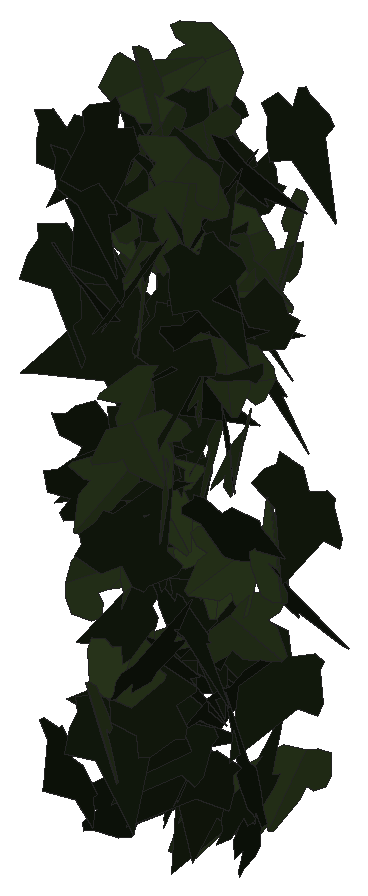
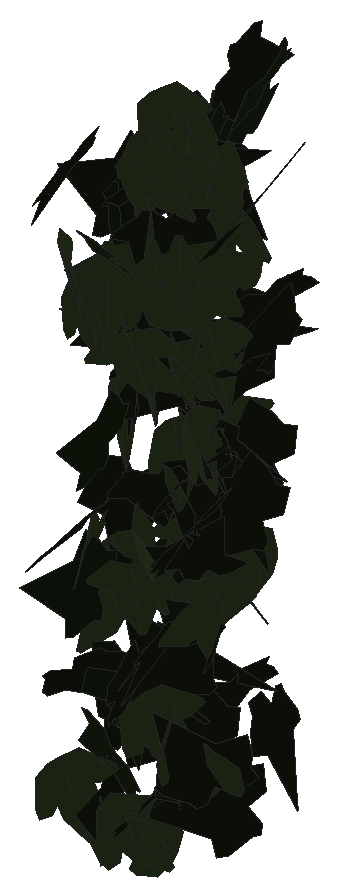
# SketchUp Ruby script. Lengths in inches.
U = 1.inch
M = Sketchup.active_model
def pt(a) = Geom::Point3d.new(a.map { |v| v * U })
def face(e, loops, mat)
  f = e.add_face(loops[0].map { |a| pt(a) })
  loops[1..].each { |l| e.add_face(l.map { |a| pt(a) }).erase! }
  f.material = f.back_material = mat if mat
  f
end
# faces: each face lists its corners as indices into pts; further lists are holes
def faces(e, pts, list, mat = nil) = list.each { |f| face(e, (f[0].is_a?(Array) ? f : [f]).map { |l| l.map { |i| pts[i] } }, mat) }
# xy, xz, yz: faces in a plane at the given z, y or x. An outline is a flat list of corners, or four numbers for a rectangle; further outlines are holes
def ring(l) = l.size == 4 ? [[l[0], l[1]], [l[2], l[1]], [l[2], l[3]], [l[0], l[3]]] : l.each_slice(2).to_a
def flat(e, list, mat, &to3) = list.each { |f| face(e, (f[0].is_a?(Array) ? f : [f]).map { |l| ring(l).map { |u, v| to3.(u, v) } }, mat) }
def xy(e, z, list, mat = nil) = flat(e, list, mat) { |x, y| [x, y, z] }
def xz(e, y, list, mat = nil) = flat(e, list, mat) { |x, z| [x, y, z] }
def yz(e, x, list, mat = nil) = flat(e, list, mat) { |y, z| [x, y, z] }
def lines(e, pts, list) = list.each { |a, b| e.add_line(pt(pts[a]), pt(pts[b])) }
# prism: a flat outline (further loops are holes) pulled along v
def prism(e, loops, v, mat = nil)
  f = face(e, loops, mat); d = Geom::Vector3d.new(v.map { |x| x * U })
  f.pushpull(f.normal.samedirection?(d) ? d.length : -d.length)
end
def box(e, o, s, mat = nil) = prism(e, [[o, [o[0] + s[0], o[1], o[2]], [o[0] + s[0], o[1] + s[1], o[2]], [o[0], o[1] + s[1], o[2]]]], [0, 0, s[2]], mat)
def at(x, y, z, deg = 0) = Geom::Transformation.translation(pt([x, y, z])) * Geom::Transformation.rotation(ORIGIN, Z_AXIS, deg.degrees)
def axes(o, x, y, z) = Geom::Transformation.new([*x, 0, *y, 0, *z, 0, *pt(o).to_a, 1])
def part(name) = M.definitions.add(name)
# library, detail: a bought-in or finely detailed component or shape, given as its bounding box
def library(name, o, s) = part(name).tap { |d| box(d.entities, o, s) }
def detail(e, o, s) = box(e.add_group.entities, o, s)
def put(e, d, t, mat = nil) = e.add_instance(d, t).tap { |i| i.material = mat if mat }
def group(e, t, mat = nil) = e.add_group.tap { |g| g.transformation = t; g.material = mat if mat }.entities
root = M.entities
M.materials.add("efeu1").color = [18, 25, 13]
M.materials.add("efeu2").color = [43, 57, 29]
c1 = part("ivyleaf_10")
p = [[0,0.5,-0.03],[-0.0625,2.02,-0.43],[-0.19,2.01,-0.46],[-0.54,1.05,-0.29],[-0.52,0.625,-0.18],[-0.83,0.76,-0.28],
  [-1.16,0.64,-0.33],[-1.15,0.33,-0.24],[-0.77,-0.39,0.02],[-0.3,-0.51,0.16],[0.04,-0.48,0.23],[-0.02,2.01,-0.4375],
  [-0.06,2.01,-0.43],[0.04,-0.49,0.23],[0.67,-0.49,0.14],[1.38,0.36,-0.2],[1.375,0.51,-0.24],[0.81,0.65,-0.19],
  [0.62,0.59,-0.15],[0.6,1.09,-0.28],[0.5,1.23,-0.31]]
faces(c1.entities,p,[[0,1,2,3,4,5,6,7,8,9,10],[11,12,0,13,14,15,16,17,18,19,20]],"efeu2")
c2 = part("ivyleaf_9")
p = [[1.54,2.16,1.25],[1.36,2.04,1.19],[-0.21,0.99,0.68],[-0.71,1.11,0.82],[-0.85,0.86,0.67],[-0.8,0.17,0.21],
  [-0.9,-0.01,0.1],[-0.67,-0.16,-0.02],[-0.08,-0.08,-0.05],[-0.03,-0.6,-0.4],[0.65,-0.88,-0.66],[0.83,-0.6,-0.49],
  [1.29,-0.42,-0.43],[1.8125,-0.07,-0.26],[1.21,0.44,0.15]]
faces(c2.entities,p,[[0,1,2,3,4,5,6,7,8,9,10,11,12,13,14]],"efeu1")
put(root,c1,axes([35.83,221.91,226.625],[-0.01925,-0.10723,-0.48799],[0.11516,0.47425,-0.10876],[0.48618,-0.11658,0.00644]))
put(root,c2,axes([35.71,221.96,223.92],[-0.21049,-0.06879,0.44829],[0.44598,0.05846,0.21837],[-0.08246,0.49178,0.03674]))
put(root,c1,axes([36.2,222,230.33],[0.03512,-0.04163,-0.49702],[-0.38979,0.30857,-0.05339],[0.31117,0.39122,-0.01078]))
put(root,c2,axes([36.14,220.125,224.125],[0.1485,0.0757,-0.4714],[-0.46854,-0.07179,-0.15912],[-0.09178,0.48899,0.04962]))
put(root,c1,axes([35.88,222.14,229.34],[0.1571,-0.45068,0.14901],[0.04345,-0.14265,-0.47725],[0.47268,0.1629,-0.00566]))
put(root,c2,axes([35.48,221.26,227.81],[0.19653,-0.05142,0.45687],[0.44624,-0.09824,-0.20302],[0.11064,0.48755,0.00728]))
put(root,c2,axes([35.78,220.73,230.93],[-0.05063,-0.49072,-0.08142],[0.00987,0.08084,-0.49332],[0.49733,-0.05156,0.0015]))
put(root,c2,axes([35.57,220.79,230.32],[0.11961,-0.19912,0.44277],[0.29411,-0.33309,-0.22924],[0.38626,0.31528,0.03744]))
put(root,c1,axes([35.96,221.6,230.47],[0.02139,-0.49578,0.06119],[0.02614,-0.06005,-0.49569],[0.49886,0.0244,0.02335]))
put(root,c1,axes([35.71,221.99,224.29],[0.4394,0.08355,0.22349],[0.22096,0.03427,-0.44722],[-0.09005,0.49178,-0.0068]))
put(root,c1,axes([35.9375,222.46,231.4],[-0.17757,-0.45325,-0.11415],[-0.0425,-0.10595,0.48679],[-0.46547,0.18259,-0.0009]))
put(root,c2,axes([35.77,220.53,232.64],[0.18937,-0.46258,0.01271],[0.00648,-0.01108,-0.49984],[0.46271,0.18947,0.0018]))
put(root,c2,axes([35.85,221.3,229.92],[0.06218,-0.43678,-0.23528],[-0.01354,0.23554,-0.44084],[0.49593,0.0612,0.01746]))
put(root,c1,axes([36,220.93,226.55],[0.0661,-0.11066,0.4831],[-0.05284,0.48303,0.11787],[-0.49279,-0.06664,0.05216]))
put(root,c2,axes([36.02,221.46,228.1],[0.00869,-0.05801,0.49655],[0.20366,0.45396,0.04947],[-0.45656,0.20139,0.03152]))
put(root,c1,axes([36.09,222.24,229.28],[-0.11377,-0.48538,-0.03829],[0.00888,0.03725,-0.49853],[0.4868,-0.11412,0.00015]))
put(root,c1,axes([35.97,221.15,231.5],[0.1612,0.43329,0.19045],[0.07558,0.17504,-0.46222],[-0.46723,0.17781,-0.00907]))
put(root,c2,axes([36.35,221.82,227],[-0.42612,-0.25663,0.05063],[0.04573,0.02221,0.49741],[-0.25755,0.42854,0.00454]))
put(root,c1,axes([36.14,220.35,226.55],[0.02203,0.06216,0.49563],[-0.10546,0.48551,-0.0562],[-0.48826,-0.10206,0.0345]))
put(root,c2,axes([36.36,221.26,228.7],[-0.03489,0.22501,0.44515],[-0.10822,0.43219,-0.22694],[-0.4869,-0.11218,0.01854]))
put(root,c2,axes([36.36,220.81,228],[-0.26637,0.41003,-0.1045],[0.0617,-0.08453,-0.48893],[-0.41862,-0.27336,-0.00556]))
put(root,c2,axes([35.98,222.03,228.58],[0.09815,-0.4821,-0.08914],[-0.02083,0.08673,-0.49198],[0.48983,0.10029,-0.00306]))
put(root,c1,axes([35.95,221.53,232.8],[-0.14964,-0.24048,0.41204],[0.25271,0.32632,0.28223],[-0.40466,0.29272,0.02388]))
put(root,c1,axes([36.57,220.62,231.88],[-0.11858,0.02557,0.48506],[-0.48569,0.00016,-0.11875],[-0.00622,-0.49935,0.0248]))
put(root,c2,axes([36.37,222.18,227.18],[-0.03373,-0.49731,0.03928],[0.00363,0.03912,0.49845],[-0.49885,0.03391,0.00097]))
put(root,c2,axes([36.3,221.75,228.3125],[-0.24248,0.17327,-0.40147],[0.25244,-0.31938,-0.2903],[-0.35704,-0.34348,0.06741]))
put(root,c1,axes([36.27,221.57,231.24],[-0.30134,-0.37153,-0.14547],[0.10367,0.10312,-0.47814],[0.38529,-0.31833,0.01488]))
put(root,c2,axes([35.98,220.94,223.02],[0.25306,0.1117,0.41651],[0.37555,0.18027,-0.27652],[-0.21194,0.4528,0.00734]))
put(root,c1,axes([36.09,222.51,224.47],[-0.08167,0.05422,0.4903],[0.31159,-0.37961,0.09388],[0.38242,0.32087,0.02822]))
put(root,c1,axes([36.45,222.37,224.94],[-0.24223,-0.37323,0.2281],[-0.12447,-0.19114,-0.44494],[0.41932,-0.27234,-0.00032]))
put(root,c2,axes([36.25,222.56,228.77],[-0.2099,-0.43479,-0.12998],[0.05211,0.11917,-0.48279],[0.4508,-0.21623,-0.00471]))
put(root,c2,axes([36.19,222.25,226.28],[0.22812,-0.36097,-0.26012],[-0.11611,0.23389,-0.4264],[0.42951,0.25494,0.02289]))
put(root,c1,axes([36.37,222.66,231.75],[-0.13228,-0.34541,0.33645],[0.059,-0.35785,-0.34418],[0.47856,-0.05135,0.13543]))
put(root,c2,axes([36.57,220.73,229.95],[-0.29236,-0.18832,0.35925],[-0.27573,-0.23252,-0.34628],[0.29748,-0.40059,0.03211]))
put(root,c2,axes([36.19,221.59,231.7],[0.03453,-0.48044,0.13409],[0.02072,-0.13292,-0.48156],[0.49838,0.03882,0.01072]))
put(root,c1,axes([36.26,221.38,233.38],[-0.33481,0.2776,-0.24665],[0.15182,-0.20075,-0.43203],[-0.3389,-0.36419,0.05014]))
put(root,c1,axes([36.68,222.29,233.29],[0.30042,-0.01225,-0.39949],[-0.39556,0.06243,-0.29939],[0.05722,0.49594,0.02782]))
put(root,c2,axes([36.28,222.26,232.5625],[-0.12659,-0.39339,-0.28145],[0.0759,0.27118,-0.41316],[0.47772,-0.14733,-0.00894]))
put(root,c1,axes([36.25,222.55,232.4],[0.2892,-0.19812,0.35653],[0.33874,-0.12679,-0.34522],[0.2272,0.44122,0.06089]))
put(root,c1,axes([36.33,221.19,230.56],[0.31818,-0.18633,0.3377],[0.28237,-0.18569,-0.36849],[0.26274,0.42521,-0.01294]))
put(root,c1,axes([36.48,221.38,227.5],[0.04237,0.46195,0.18658],[0.01995,0.18553,-0.46388],[-0.4978,0.04675,-0.00271]))
put(root,c1,axes([36.57,220.79,226.47],[0.03032,-0.03031,-0.49816],[0.09243,0.49078,-0.02424],[0.49045,-0.09062,0.03537]))
put(root,c2,axes([36.25,220.07,227.88],[0.20836,0.03603,0.45309],[0.44505,0.08505,-0.21142],[-0.0923,0.49139,0.00338]))
put(root,c2,axes([36.46,220.64,224.62],[0.00523,-0.48569,-0.11864],[0.00219,0.11867,-0.48571],[0.49997,0.00456,0.00336]))
put(root,c2,axes([36.22,221.32,224.08],[0.26163,-0.02888,0.42511],[0.42358,-0.03643,-0.26316],[0.04618,0.49783,0.0054]))
put(root,c1,axes([36.49,222.53,227.74],[0.22776,-0.25459,0.36511],[0.22721,-0.28618,-0.34129],[0.38275,0.32138,-0.01467]))
put(root,c2,axes([37,220.71,228.46],[-0.47125,-0.00985,0.1668],[-0.16684,0.00021,-0.47134],[0.00922,-0.4999,-0.00348]))
put(root,c1,axes([36.85,220.29,228.36],[-0.16351,-0.36941,0.29463],[-0.12626,-0.26627,-0.40393],[0.45533,-0.20649,-0.00621]))
put(root,c1,axes([36.67,222.51,230.64],[0.39902,0.28378,-0.10127],[-0.07346,-0.07135,-0.4894],[-0.29221,0.40544,-0.01524]))
put(root,c1,axes([36.54,221.17,228.48],[-0.14806,0.18117,0.44188],[0.2917,-0.33199,0.23386],[0.37814,0.32704,-0.00739]))
put(root,c1,axes([36.7,221.2,231.4],[-0.06066,0.19349,-0.45704],[-0.04518,-0.46068,-0.18904],[-0.49425,0.01836,0.07337]))
put(root,c1,axes([36.97,221.78,229.92],[0.30797,0.11733,0.37602],[-0.35523,-0.12349,0.32948],[0.17019,-0.47009,0.0073]))
put(root,c1,axes([36.72,221.74,222.52],[0.07657,-0.39568,0.29593],[-0.04578,0.2925,0.40293],[-0.49198,-0.0888,0.00857]))
put(root,c2,axes([37.15,221.82,230.46],[-0.16006,0.10403,0.46212],[-0.36608,0.2824,-0.19036],[-0.30061,-0.39929,-0.01423]))
put(root,c2,axes([37.18,220.8,224.96],[-0.35881,0.09742,0.33431],[-0.32734,0.06932,-0.37154],[-0.11874,-0.48549,0.01404]))
put(root,c2,axes([36.95,221.2,223.44],[0.01115,0.20605,0.45543],[-0.02854,0.45506,-0.20519],[-0.49906,-0.02142,0.02191]))
put(root,c1,axes([36.85,220.92,232.61],[0.30665,-0.38989,-0.06284],[-0.03156,0.05512,-0.49595],[0.39366,0.30814,0.0092]))
put(root,c1,axes([37.14,222.32,222.99],[-0.22968,-0.13438,0.42331],[-0.35218,-0.23524,-0.26576],[0.27059,-0.42024,0.01341]))
put(root,c2,axes([37.02,220.65,232.45],[-0.07166,0.25255,-0.42554],[-0.00967,-0.43061,-0.25394],[-0.49474,-0.02817,0.0666]))
put(root,c2,axes([37.15,220.38,226.53],[-0.40754,0.27429,0.09315],[-0.07777,0.05128,-0.49125],[-0.27904,-0.41489,0.00087]))
put(root,c2,axes([36.8,222.14,223.17],[-0.12397,-0.43608,0.21086],[-0.03416,-0.20925,-0.45282],[0.48318,-0.12668,0.02208]))
put(root,c2,axes([36.57,221.5,224.86],[0.42777,0.24655,-0.07889],[0.06752,0.04084,0.49373],[0.24991,-0.43306,0.00164]))
put(root,c2,axes([37.11,221.28,224.43],[-0.49992,-0.00754,-0.00471],[0.00471,-0.00007,-0.49998],[0.00754,-0.49994,0.00014]))
put(root,c1,axes([36.85,220.19,225.47],[0.16212,0.3791,-0.28284],[0.11055,0.26035,0.41231],[0.45989,-0.19623,0.0006]))
put(root,c2,axes([36.69,221.91,223.35],[0.03922,-0.43058,0.25112],[0.065,-0.24533,-0.4308],[0.4942,0.06644,0.03674]))
put(root,c1,axes([37.01,220.61,229.56],[-0.12029,-0.4666,0.13349],[-0.03388,-0.12912,-0.48185],[0.48413,-0.12497,-0.00055]))
put(root,c2,axes([36.72,221.97,225.6875],[0.16002,-0.47148,0.04579],[0.00717,-0.04592,-0.49784],[0.47365,0.15999,-0.00794]))
put(root,c1,axes([36.97,221.23,230.58],[0.33998,-0.32611,0.16753],[-0.12489,0.11179,0.47107],[-0.3447,-0.36215,-0.00545]))
put(root,c2,axes([36.86,221.75,230.16],[-0.09527,-0.48221,-0.09166],[0.02616,0.08825,-0.49145],[0.49014,-0.09844,0.00842]))
put(root,c2,axes([37.22,221.125,224.09],[0.11165,0.20978,-0.43992],[-0.21567,-0.38345,-0.23759],[-0.43706,0.24281,0.00486]))
put(root,c2,axes([37.01,222.37,224.99],[-0.04707,-0.11607,0.48406],[-0.17941,-0.44958,-0.12525],[0.46432,-0.18548,0.00068]))
put(root,c2,axes([36.8,220.83,225.61],[0.49909,-0.00608,-0.02961],[-0.02953,0.00633,-0.49909],[0.00644,0.49992,0.00596]))
put(root,c1,axes([37.05,220.75,232.96],[-0.01421,-0.45776,-0.20062],[0.02185,0.19994,-0.45776],[0.49932,-0.02178,0.01432]))
put(root,c1,axes([36.79,220.77,228.19],[-0.29871,0.03175,0.39971],[0.38056,-0.13455,0.29508],[0.1263,0.48051,0.05621]))
put(root,c2,axes([36.92,220.18,227.16],[-0.2868,-0.01503,0.40929],[0.39876,-0.12425,0.27486],[0.09345,0.48408,0.08326]))
put(root,c1,axes([37.11,222.4,231.44],[0.00857,-0.47805,-0.14625],[0.01868,0.14648,-0.4777],[0.49958,0.00272,0.02037]))
put(root,c1,axes([37,222.01,226.7],[0.44685,0.22432,-0.0017],[-0.00163,-0.00055,-0.5],[-0.22432,0.44685,0.00024]))
put(root,c2,axes([37.47,221.9,231.46],[-0.19844,0.36539,0.27769],[-0.29874,0.12682,-0.38036],[-0.34839,-0.31687,0.16798]))
put(root,c2,axes([36.82,220.78,232.77],[0.23987,-0.40791,0.16146],[0.07209,-0.14487,-0.47309],[0.43274,0.25024,-0.01069]))
put(root,c2,axes([37.47,220.74,232.23],[-0.15187,-0.02789,0.47556],[-0.46996,-0.07288,-0.15436],[0.07793,-0.49387,-0.00408]))
put(root,c2,axes([37.15,219.71,233.5],[0.00347,-0.13317,-0.48193],[0.27049,-0.40483,0.11381],[-0.42051,-0.2615,0.06923]))
put(root,c1,axes([37.51,221.89,231.22],[-0.15294,-0.15372,0.45053],[-0.31561,-0.32152,-0.21684],[0.35637,-0.35071,0.00132]))
put(root,c2,axes([37.08,221.46,232.51],[-0.05507,-0.44276,-0.22568],[0.072,0.21755,-0.44439],[0.49171,-0.08145,0.0398]))
put(root,c1,axes([37.31,221.27,232.875],[-0.16171,-0.45505,-0.12954],[0.03414,0.12532,-0.48283],[0.47189,-0.165,-0.00946]))
put(root,c1,axes([37.48,221.63,226.77],[0.37165,-0.08785,-0.32273],[-0.30779,0.099,-0.3814],[0.13091,0.48216,0.01951]))
put(root,c2,axes([37.02,219.21,233.07],[0.22816,-0.42475,0.1324],[0.06956,-0.11291,-0.48209],[0.43944,0.23841,0.00757]))
put(root,c2,axes([37.5,221.5625,224.98],[-0.04759,0.49571,-0.04479],[0.00393,-0.04462,-0.49799],[-0.49771,-0.04775,0.00035]))
put(root,c1,axes([37.32,219.98,229.2],[-0.33333,-0.33039,-0.17243],[0.12346,0.12038,-0.46933],[0.35164,-0.35546,0.00132]))
put(root,c2,axes([37.13,220.7,229.41],[0.40006,0.23957,0.18044],[0.15846,0.08656,-0.46626],[-0.25464,0.43025,-0.00666]))
put(root,c2,axes([37.04,222.6,229.02],[0.31169,-0.35101,0.17217],[0.10877,-0.13364,-0.46937],[0.37553,0.33005,-0.00695]))
put(root,c2,axes([37.58,221.41,232.11],[-0.25645,0.39398,-0.17032],[0.1029,-0.13618,-0.46996],[-0.41671,-0.2761,-0.01123]))
put(root,c1,axes([37.45,221.24,229.68],[0.19333,-0.45661,-0.06427],[-0.01692,0.06262,-0.49577],[0.4608,0.19387,0.00877]))
put(root,c2,axes([37.4,220.77,230.28],[-0.39712,-0.11505,-0.28117],[0.27781,0.04975,-0.41273],[0.12295,-0.48403,0.02441]))
put(root,c1,axes([37.21,220.68,228.26],[0.12122,-0.12219,0.46944],[0.34272,-0.32087,-0.17201],[0.3433,0.36347,0.00596]))
put(root,c1,axes([37.4,222.06,230.51],[-0.05868,0.06206,0.49265],[0.13551,-0.47525,0.07601],[0.4777,0.14244,0.03895]))
put(root,c2,axes([37.54,221.79,222.68],[0.00722,0.03182,0.49893],[0.12382,0.48333,-0.03262],[-0.48437,0.12403,-0.0009]))
put(root,c2,axes([37.35,219.89,225.78],[0.13102,0.45857,0.15017],[-0.04833,-0.14235,0.47686],[0.4801,-0.13947,0.00702]))
put(root,c2,axes([37.32,219.18,232.26],[0.32398,-0.2447,-0.29182],[0.22608,-0.18474,0.40591],[-0.30648,-0.39496,-0.00906]))
put(root,c1,axes([37.79,220.34,232.97],[-0.40163,-0.09567,0.28203],[-0.25961,-0.11956,-0.41026],[0.14593,-0.47598,0.04636]))
put(root,c2,axes([37.18,221.125,230.18],[0.21161,0.18566,-0.41322],[0.23824,0.34231,0.2758],[0.38531,-0.31362,0.05641]))
put(root,c2,axes([37.65,221.23,227.6],[0.36773,0.21135,-0.26478],[-0.24534,-0.10336,-0.42323],[-0.23363,0.44119,0.02769]))
put(root,c2,axes([37.32,221.73,230.55],[0.37801,-0.31644,0.08353],[0.06461,-0.05294,-0.49297],[0.32084,0.38349,0.00087]))
put(root,c2,axes([37.33,220.73,226.43],[0.29764,-0.38224,0.12368],[0.08276,-0.09229,-0.48439],[0.39314,0.30882,0.00834]))
put(root,c1,axes([37.76,220.375,232.51],[-0.32896,-0.36747,0.08215],[-0.04913,-0.06627,-0.49315],[0.37332,-0.33253,0.0075]))
put(root,c1,axes([37.78,222.55,223.58],[-0.21924,-0.41563,0.17084],[-0.06377,-0.15939,-0.4696],[0.44482,-0.22771,0.01688]))
put(root,c1,axes([38.0625,221.21,230],[-0.30398,0.00223,0.39698],[-0.37859,-0.15205,-0.28905],[0.11943,-0.47632,0.09412]))
put(root,c2,axes([37.85,221.41,223.4],[-0.34675,0.33255,-0.13847],[-0.10238,0.09329,0.48043],[0.34537,0.36154,0.0034]))
put(root,c2,axes([37.78,222.33,225.13],[-0.28954,-0.40148,0.07055],[-0.03984,-0.05825,-0.49499],[0.40568,-0.29226,0.00175]))
put(root,c2,axes([37.38,221.66,232.29],[0.255,-0.22216,0.36827],[0.31774,-0.19122,-0.33537],[0.28986,0.40507,0.04366]))
put(root,c1,axes([37.73,221.45,226.04],[-0.2092,-0.33645,-0.30502],[0.16243,0.25818,-0.39618],[0.42409,-0.26485,0.00128]))
put(root,c1,axes([37.85,222.125,230.85],[0.00822,-0.48851,0.10626],[0.01714,-0.10594,-0.48835],[0.49964,0.01167,0.015]))
put(root,c2,axes([37.66,220.92,230.14],[0.43551,0.19977,0.14289],[-0.12875,-0.06203,0.47914],[0.20917,-0.45414,-0.00259]))
put(root,c2,axes([38.26,221.16,230.22],[-0.15289,0.19,0.43649],[-0.42838,0.14507,-0.21319],[-0.20765,-0.43915,0.11842]))
put(root,c1,axes([37.74,218.61,226.16],[-0.28763,0.32565,-0.24743],[0.16914,-0.1807,-0.43444],[-0.37238,-0.33361,-0.00621]))
put(root,c1,axes([37.51,221.67,230.85],[0.04154,-0.05857,0.49482],[0.49793,0.02333,-0.03904],[-0.01852,0.49601,0.06026]))
put(root,c1,axes([37.96,221.15,228.81],[0.12756,-0.46739,-0.12361],[-0.03455,0.11869,-0.48448],[0.48222,0.13214,-0.00202]))
put(root,c2,axes([37.76,222.75,227.27],[-0.07177,-0.43998,0.22641],[0.03831,-0.23304,-0.44071],[0.49334,-0.04592,0.06716]))
put(root,c1,axes([37.99,220.88,230.17],[-0.47025,-0.16877,0.01944],[-0.01831,-0.00654,-0.49962],[0.1689,-0.47061,-0.00003]))
put(root,c1,axes([38.04,221.75,226.59],[-0.11226,0.42059,-0.24596],[-0.09143,0.22974,0.43458],[0.47858,0.14255,0.02533]))
put(root,c2,axes([37.71,221.21,228.66],[-0.02005,0.01021,0.49949],[0.09031,-0.49159,0.01368],[0.49137,0.09076,0.01787]))
put(root,c2,axes([38.1875,218.88,232.14],[-0.26908,0.41834,-0.0509],[0.02848,-0.0422,-0.4974],[-0.42046,-0.27058,-0.00111]))
put(root,c1,axes([37.95,222.32,231.45],[0.33359,-0.36957,0.04625],[0.03,-0.03522,-0.49785],[0.37124,0.33493,-0.00132]))
put(root,c2,axes([37.78,220.62,231.52],[0.18991,-0.42077,-0.19206],[-0.04521,0.18974,-0.46038],[0.46032,0.19223,0.03402]))
put(root,c2,axes([38.17,221.17,223.76],[0.10938,-0.21037,0.44021],[-0.15085,0.41444,0.23554],[-0.46398,-0.18434,0.0272]))
put(root,c2,axes([37.6,222.14,226.33],[0.35667,-0.2236,0.26979],[0.2316,-0.13845,-0.42094],[0.26295,0.42524,0.00481]))
put(root,c2,axes([37.92,222.29,232.92],[0.21944,-0.42612,-0.14237],[-0.07563,0.12115,-0.47917],[0.44286,0.23183,-0.01128]))
